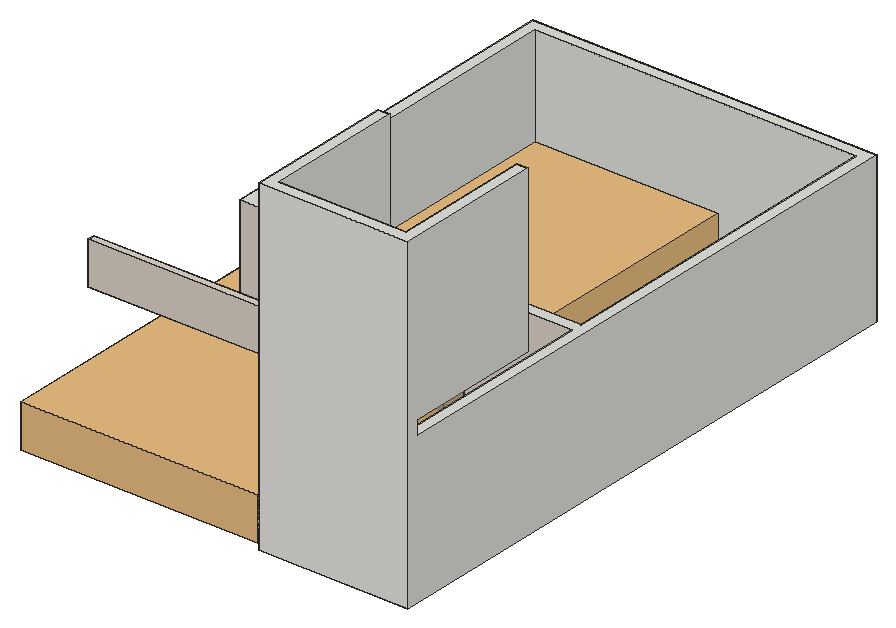
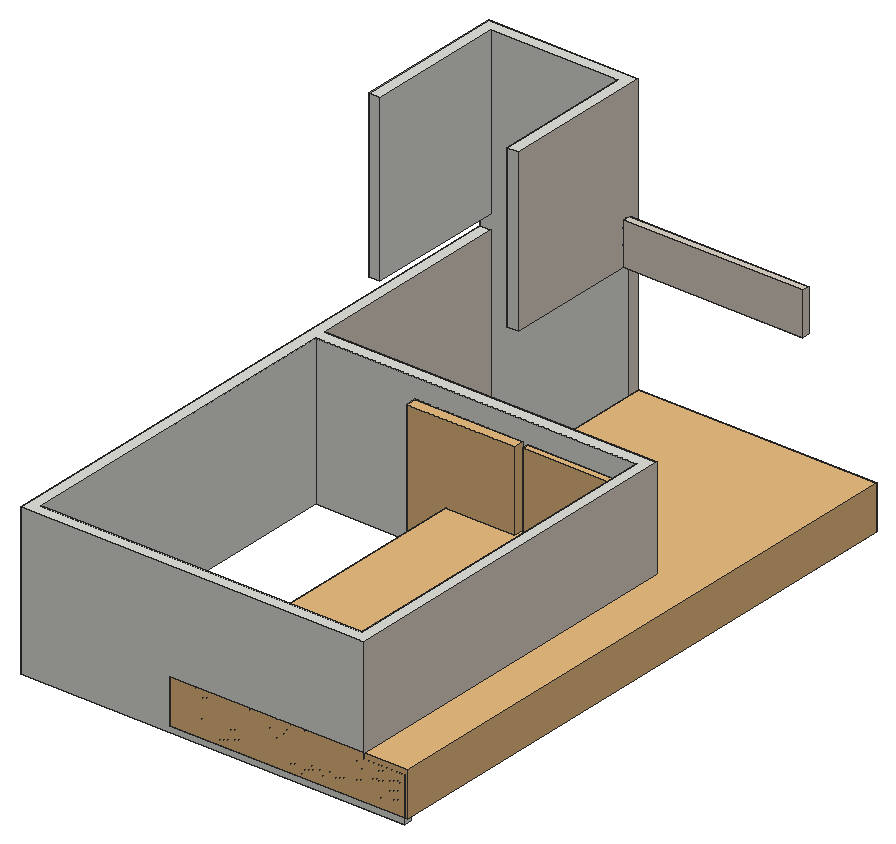
# SketchUp Ruby script. Lengths in inches.
U = 1.inch
M = Sketchup.active_model
def pt(a) = Geom::Point3d.new(a.map { |v| v * U })
def face(e, loops, mat)
  f = e.add_face(loops[0].map { |a| pt(a) })
  loops[1..].each { |l| e.add_face(l.map { |a| pt(a) }).erase! }
  f.material = f.back_material = mat if mat
  f
end
# faces: each face lists its corners as indices into pts; further lists are holes
def faces(e, pts, list, mat = nil) = list.each { |f| face(e, (f[0].is_a?(Array) ? f : [f]).map { |l| l.map { |i| pts[i] } }, mat) }
# xy, xz, yz: faces in a plane at the given z, y or x. An outline is a flat list of corners, or four numbers for a rectangle; further outlines are holes
def ring(l) = l.size == 4 ? [[l[0], l[1]], [l[2], l[1]], [l[2], l[3]], [l[0], l[3]]] : l.each_slice(2).to_a
def flat(e, list, mat, &to3) = list.each { |f| face(e, (f[0].is_a?(Array) ? f : [f]).map { |l| ring(l).map { |u, v| to3.(u, v) } }, mat) }
def xy(e, z, list, mat = nil) = flat(e, list, mat) { |x, y| [x, y, z] }
def xz(e, y, list, mat = nil) = flat(e, list, mat) { |x, z| [x, y, z] }
def yz(e, x, list, mat = nil) = flat(e, list, mat) { |y, z| [x, y, z] }
def lines(e, pts, list) = list.each { |a, b| e.add_line(pt(pts[a]), pt(pts[b])) }
# prism: a flat outline (further loops are holes) pulled along v
def prism(e, loops, v, mat = nil)
  f = face(e, loops, mat); d = Geom::Vector3d.new(v.map { |x| x * U })
  f.pushpull(f.normal.samedirection?(d) ? d.length : -d.length)
end
def box(e, o, s, mat = nil) = prism(e, [[o, [o[0] + s[0], o[1], o[2]], [o[0] + s[0], o[1] + s[1], o[2]], [o[0], o[1] + s[1], o[2]]]], [0, 0, s[2]], mat)
def at(x, y, z, deg = 0) = Geom::Transformation.translation(pt([x, y, z])) * Geom::Transformation.rotation(ORIGIN, Z_AXIS, deg.degrees)
def axes(o, x, y, z) = Geom::Transformation.new([*x, 0, *y, 0, *z, 0, *pt(o).to_a, 1])
def part(name) = M.definitions.add(name)
# library, detail: a bought-in or finely detailed component or shape, given as its bounding box
def library(name, o, s) = part(name).tap { |d| box(d.entities, o, s) }
def detail(e, o, s) = box(e.add_group.entities, o, s)
def put(e, d, t, mat = nil) = e.add_instance(d, t).tap { |i| i.material = mat if mat }
def group(e, t, mat = nil) = e.add_group.tap { |g| g.transformation = t; g.material = mat if mat }.entities
root = M.entities
M.materials.add("1755 AP K184 Brass Olive-N").color = [221, 212, 201]
M.materials.add("Antracyt").color = [44, 47, 50]
M.materials.add("[0135_DarkGray]").color = [81, 81, 81]
M.materials.add("[Carrera Marble]").color = [233, 230, 225]
M.materials.add("[Metal Seamed]").color = [15, 15, 15]
M.materials.add("[Translucent Glass Gray]").color = [128, 128, 128]
M.materials["[Translucent Glass Gray]"].alpha = 0.15
c1 = library("Group\#24",[0,0,0],[191,470.5,35])
c2 = part("หน้าต่าง3บาน")
xy(c2.entities,42.78,[[77.6875,12.74,148.55,16.68]],"Antracyt")
xy(c2.entities,43.96,[[78.87,12.74,147.37,12.74,147.37,14.71,125.72,14.71,125.72,13.13,100.52,13.13,100.52,14.71,78.87,14.71],[100.52,13.13,102.88,14.71],[123.36,13.13,125.72,14.71],[102.49,14.71,123.75,14.71,123.75,16.28,147.37,16.28,147.37,16.68,78.87,16.68,78.87,16.28,102.49,16.28]],"Antracyt")
xy(c2.entities,45.93,[[102.49,13.13,123.75,13.92],[102.49,13.92,123.75,14.71],[80.84,14.71,100.52,15.49],[125.72,14.71,145.4,15.49],[80.84,15.49,100.52,16.28],
  [125.72,15.49,145.4,16.28]],"Antracyt")
xy(c2.entities,83.09,[[102.49,13.13,123.75,13.92],[102.49,13.92,123.75,14.71],[80.84,14.71,100.52,15.49],[125.72,14.71,145.4,15.49],[80.84,15.49,100.52,16.28],
  [125.72,15.49,145.4,16.28]],"Antracyt")
xy(c2.entities,84.91,[[78.87,12.74,78.87,14.71,100.52,14.71,100.52,13.13,125.72,13.13,125.72,14.71,147.37,14.71,147.37,12.74],[100.52,13.13,125.72,14.71],[102.49,14.71,102.49,16.28,78.87,16.28,78.87,16.68,147.37,16.68,147.37,16.28,123.75,16.28,123.75,14.71],[78.87,14.71,102.49,16.28]],"Antracyt")
xy(c2.entities,86.09,[[77.6875,12.74,148.55,16.68]],"Antracyt")
xz(c2.entities,12.74,[[[77.6875,42.78,148.55,86.09],[78.87,43.96,147.37,84.91]]],"Antracyt")
xz(c2.entities,13.13,[[[100.52,43.96,125.72,84.91],[102.49,45.93,123.75,83.09]]],"Antracyt")
xz(c2.entities,13.92,[[102.49,45.93,123.75,83.09]],"Antracyt")
xz(c2.entities,14.71,[[78.87,43.96,100.52,43.96,100.52,45.93,80.84,45.93,80.84,83.09,100.52,83.09,100.52,84.91,78.87,84.91],[100.52,43.96,102.49,84.91],[102.49,43.96,123.75,45.93],[125.72,43.96,147.37,43.96,147.37,84.91,125.72,84.91,125.72,83.09,145.4,83.09,145.4,45.93,125.72,45.93],[102.49,83.09,123.75,84.91]],"Antracyt")
xz(c2.entities,15.49,[[80.84,45.93,100.52,83.09],[125.72,45.93,145.4,83.09],[80.44,82.9375,80.84,83.73]],"Antracyt")
xz(c2.entities,16.28,[[[78.87,43.96,102.49,84.91],[80.84,45.93,100.52,83.09]],[[123.75,43.96,147.37,84.91],[125.72,45.93,145.4,83.09]]],"Antracyt")
xz(c2.entities,16.68,[[[77.6875,42.78,148.55,86.09],[78.87,43.96,147.37,84.91]]],"Antracyt")
yz(c2.entities,77.6875,[[12.74,42.78,16.68,86.09]],"Antracyt")
yz(c2.entities,78.87,[[12.74,43.96,14.71,84.91],[16.28,43.96,16.68,84.91]],"Antracyt")
yz(c2.entities,80.84,[[14.71,45.93,15.49,83.09],[15.49,45.93,16.28,83.09]],"Antracyt")
yz(c2.entities,100.52,[[13.13,43.96,14.71,84.91],[14.71,45.93,15.49,83.09],[15.49,45.93,16.28,83.09]],"Antracyt")
yz(c2.entities,102.49,[[14.71,43.96,16.28,84.91],[13.13,45.93,13.92,83.09],[13.92,45.93,14.71,83.09]],"Antracyt")
yz(c2.entities,123.75,[[14.71,43.96,16.28,84.91],[13.13,45.93,13.92,83.09],[13.92,45.93,14.71,83.09]],"Antracyt")
yz(c2.entities,125.72,[[13.13,43.96,14.71,84.91],[14.71,45.93,15.49,83.09],[15.49,45.93,16.28,83.09]],"Antracyt")
yz(c2.entities,145.4,[[14.71,45.93,15.49,83.09],[15.49,45.93,16.28,83.09]],"Antracyt")
yz(c2.entities,147.37,[[12.74,43.96,14.71,84.91],[16.28,43.96,16.68,84.91]],"Antracyt")
yz(c2.entities,148.55,[[12.74,42.78,16.68,86.09]],"Antracyt")
p = [[80.44,15.49,84.91],[80.44,15.49,83.73]]
lines(c2.entities,p,[[0,1]])
c3 = part("PENTEK_RP Fineline 50S_Sliding_DoorCase_E1")
box(c3.entities,[0,0,0],[1.51,3.66,99.27],"[0135_DarkGray]")
c4 = part("PENTEK_RP Fineline 50S_SlidingDooe_Case_E2")
box(c4.entities,[0,0,0],[96.25,3.66,1.51],"[0135_DarkGray]")
c5 = part("pentek_RP Fineline 50S_SlidingDoor_Case")
put(c5.entities,c3,at(97.76,0,0))
put(c5.entities,c4,at(1.51,0,0))
put(c5.entities,c3,at(0,0,0))
put(c5.entities,c4,at(1.51,0,97.76))
c6 = part("PENTEK_RP Fineline 50S_SlidingDoor_GlazingBead_2")
box(c6.entities,[0,0,0],[0.56,0.59,94.39],"[0135_DarkGray]")
c7 = part("PENTEK_RP Fineline 50S_SlidingDoor_Glass")
box(c7.entities,[0,0,0],[46.58,0.16,94.39],"[Translucent Glass Gray]")
c8 = part("PENTEK_RP Fineline 50S_SlidingDoor_GlazingBead")
box(c8.entities,[0,0,0],[45.47,0.59,0.56],"[0135_DarkGray]")
c9 = part("PENTEK_RP Fineline 50S_SlidingDoor_Leaf_E1")
xy(c9.entities,0,[[0,0,0.93,1.97],[0.93,1.57,1.49,1.97]],"[0135_DarkGray]")
xy(c9.entities,96.25,[[0,0,0.93,0,0.93,1.57,1.49,1.57,1.49,1.97,0,1.97]],"[0135_DarkGray]")
xz(c9.entities,0,[[0,0,0.93,96.25]],"[0135_DarkGray]")
xz(c9.entities,1.57,[[0.93,0,1.49,95.32],[0.93,95.32,1.49,96.25]],"[0135_DarkGray]")
xz(c9.entities,1.97,[[0,0,1.49,96.25]],"[0135_DarkGray]")
yz(c9.entities,0,[[0,0,1.97,96.25]],"[0135_DarkGray]")
yz(c9.entities,0.93,[[0,0,1.57,0.93],[0,0.93,1.57,95.32],[0,95.32,1.57,96.25]],"[0135_DarkGray]")
yz(c9.entities,1.49,[[1.57,0,1.97,95.32],[1.57,95.32,1.97,96.25]],"[0135_DarkGray]")
c10 = part("PENTEK_RP Fineline 50S_SlidingDoor_Leaf_E2")
xy(c10.entities,0,[[0,0,0,1.57,0.56,1.57,0.56,1.97,46.02,1.97,46.02,1.57,46.58,1.57,46.58,0]],"[0135_DarkGray]")
xy(c10.entities,0.93,[[0,0,46.58,1.57]],"[0135_DarkGray]")
xy(c10.entities,1.49,[[0.56,1.57,46.02,1.97]],"[0135_DarkGray]")
xz(c10.entities,0,[[0,0,46.58,0.93]],"[0135_DarkGray]")
xz(c10.entities,1.57,[[0,0,0.56,0.93],[46.02,0,46.58,0.93],[0.56,0.93,46.02,1.49]],"[0135_DarkGray]")
xz(c10.entities,1.97,[[0.56,0,46.02,1.49]],"[0135_DarkGray]")
yz(c10.entities,0,[[0,0,1.57,0.93]],"[0135_DarkGray]")
yz(c10.entities,0.56,[[1.57,0,1.97,0.93],[1.57,0.93,1.97,1.49]],"[0135_DarkGray]")
yz(c10.entities,46.02,[[1.57,0,1.97,0.93],[1.57,0.93,1.97,1.49]],"[0135_DarkGray]")
yz(c10.entities,46.58,[[0,0,1.57,0.93]],"[0135_DarkGray]")
c11 = part("PENTEK_RP Fineline S_SlidingDoor_Leaf1")
put(c11.entities,c6,at(0.93,0,0.93))
put(c11.entities,c6,at(46.96,0,0.93))
put(c11.entities,c7,at(1.49,1.42,0.93))
put(c11.entities,c8,at(1.49,0,0.93))
put(c11.entities,c7,at(1.49,0.59,0.93))
put(c11.entities,c9,at(0,0,0))
put(c11.entities,c9,axes([48.44,0,0],[-1,0,0],[0,1,0],[0,0,1]))
put(c11.entities,c10,axes([0.93,0,96.25],[1,0,0],[0,1,0],[0,0,-1]))
put(c11.entities,c10,at(0.93,0,0))
put(c11.entities,c8,at(1.49,0,94.77))
c12 = part("PENTEK_RP Fineline 50S_SlidingDoor_Leaf2")
put(c12.entities,c7,at(1.49,1.42,0.93))
put(c12.entities,c8,at(1.49,0,94.77))
put(c12.entities,c6,at(46.96,0,0.93))
put(c12.entities,c7,at(1.49,0.59,0.93))
put(c12.entities,c6,at(0.93,0,0.93))
put(c12.entities,c9,at(0,0,0))
put(c12.entities,c9,axes([48.44,0,0],[-1,0,0],[0,1,0],[0,0,1]))
put(c12.entities,c8,at(1.49,0,0.93))
put(c12.entities,c10,axes([0.93,0,96.25],[1,0,0],[0,1,0],[0,0,-1]))
put(c12.entities,c10,at(0.93,0,0))
c13 = part("PENTEK_RP+Fineline+50S_Sliding_Door (1)")
put(c13.entities,c5,at(0,-1.88,-0.09))
put(c13.entities,c11,at(1.51,-2.27,1.42))
put(c13.entities,c12,at(49.32,-0.3,1.42))
c14 = library("Untitled",[23.5,7.18,0],[66.61,8.2,79.03])
xy(root,132,[[30.34,172.75,30.26,172.76,30.1875,172.77,30.11,172.78,29.95,172.8,29.875,172.82,29.8,172.83,29.72,172.85,29.65,172.875,29.57,172.9,29.5,172.92,29.42,172.95,29.21,173.04,29.14,173.08,29.07,173.11,28.93,173.19,28.87,173.23,28.8,173.28,28.74,173.32,28.67,173.37,28.43,173.57,28.38,173.63,28.32,173.68,28.12,173.92,28.07,173.99,28.03,174.05,27.98,174.12,27.94,174.18,27.86,174.32,27.83,174.39,27.79,174.46,27.7,174.67,27.67,174.75,27.65,174.82,27.625,174.9,27.6,174.97,27.58,175.05,27.57,175.125,27.55,175.2,27.53,175.36,27.52,175.4375,27.51,175.51,27.5,175.59,27.5,175.91,27.51,175.99,27.52,176.0625,27.53,176.14,27.55,176.3,27.57,176.375,27.58,176.45,27.6,176.53,27.625,176.6,27.65,176.68,27.67,176.75,27.7,176.83,27.79,177.04,27.83,177.11,27.86,177.18,27.94,177.32,27.98,177.38,28.03,177.45,28.07,177.51,28.12,177.58,28.32,177.82,28.38,177.87,28.43,177.93,28.67,178.13,28.74,178.18,28.8,178.22,28.87,178.27,28.93,178.31,29.07,178.39,29.14,178.42,29.21,178.46,29.42,178.55,29.5,178.58,29.57,178.6,29.65,178.625,29.72,178.65,29.8,178.67,29.875,178.68,29.95,178.7,30.11,178.72,30.1875,178.73,30.26,178.74,30.34,178.75,30.66,178.75,30.74,178.74,30.8125,178.73,30.89,178.72,31.05,178.7,31.125,178.68,31.2,178.67,31.28,178.65,31.35,178.625,31.43,178.6,31.5,178.58,31.58,178.55,31.79,178.46,31.86,178.42,31.93,178.39,32.07,178.31,32.13,178.27,32.2,178.22,32.26,178.18,32.33,178.13,32.57,177.93,32.62,177.87,32.68,177.82,32.88,177.58,32.93,177.51,32.97,177.45,33.02,177.38,33.06,177.32,33.14,177.18,33.17,177.11,33.21,177.04,33.3,176.83,33.33,176.75,33.35,176.68,33.375,176.6,33.4,176.53,33.42,176.45,33.43,176.375,33.45,176.3,33.47,176.14,33.48,176.0625,33.49,175.99,33.5,175.91,33.5,175.59,33.49,175.51,33.48,175.4375,33.47,175.36,33.45,175.2,33.43,175.125,33.42,175.05,33.4,174.97,33.375,174.9,33.35,174.82,33.33,174.75,33.3,174.67,33.21,174.46,33.17,174.39,33.14,174.32,33.06,174.18,33.02,174.12,32.97,174.05,32.93,173.99,32.88,173.92,32.68,173.68,32.62,173.63,32.57,173.57,32.33,173.37,32.26,173.32,32.2,173.28,32.13,173.23,32.07,173.19,31.93,173.11,31.86,173.08,31.79,173.04,31.58,172.95,31.5,172.92,31.43,172.9,31.35,172.875,31.28,172.85,31.2,172.83,31.125,172.82,31.05,172.8,30.89,172.78,30.8125,172.77,30.74,172.76,30.66,172.75],[100.84,172.75,100.76,172.76,100.6875,172.77,100.61,172.78,100.45,172.8,100.375,172.82,100.3,172.83,100.22,172.85,100.15,172.875,100.07,172.9,100,172.92,99.92,172.95,99.71,173.04,99.64,173.08,99.57,173.11,99.43,173.19,99.37,173.23,99.3,173.28,99.24,173.32,99.17,173.37,98.93,173.57,98.88,173.63,98.82,173.68,98.62,173.92,98.57,173.99,98.53,174.05,98.48,174.12,98.44,174.18,98.36,174.32,98.33,174.39,98.29,174.46,98.2,174.67,98.17,174.75,98.15,174.82,98.125,174.9,98.1,174.97,98.08,175.05,98.07,175.125,98.05,175.2,98.03,175.36,98.02,175.4375,98.01,175.51,98,175.59,98,175.91,98.01,175.99,98.02,176.0625,98.03,176.14,98.05,176.3,98.07,176.375,98.08,176.45,98.1,176.53,98.125,176.6,98.15,176.68,98.17,176.75,98.2,176.83,98.29,177.04,98.33,177.11,98.36,177.18,98.44,177.32,98.48,177.38,98.53,177.45,98.57,177.51,98.62,177.58,98.82,177.82,98.88,177.87,98.93,177.93,99.17,178.13,99.24,178.18,99.3,178.22,99.37,178.27,99.43,178.31,99.57,178.39,99.64,178.42,99.71,178.46,99.92,178.55,100,178.58,100.07,178.6,100.15,178.625,100.22,178.65,100.3,178.67,100.375,178.68,100.45,178.7,100.61,178.72,100.6875,178.73,100.76,178.74,100.84,178.75,101.16,178.75,101.24,178.74,101.3125,178.73,101.39,178.72,101.55,178.7,101.625,178.68,101.7,178.67,101.78,178.65,101.85,178.625,101.93,178.6,102,178.58,102.08,178.55,102.29,178.46,102.36,178.42,102.43,178.39,102.57,178.31,102.63,178.27,102.7,178.22,102.76,178.18,102.83,178.13,103.07,177.93,103.12,177.87,103.18,177.82,103.38,177.58,103.43,177.51,103.47,177.45,103.52,177.38,103.56,177.32,103.64,177.18,103.67,177.11,103.71,177.04,103.8,176.83,103.83,176.75,103.85,176.68,103.875,176.6,103.9,176.53,103.92,176.45,103.93,176.375,103.95,176.3,103.97,176.14,103.98,176.0625,103.99,175.99,104,175.91,104,175.59,103.99,175.51,103.98,175.4375,103.97,175.36,103.95,175.2,103.93,175.125,103.92,175.05,103.9,174.97,103.875,174.9,103.85,174.82,103.83,174.75,103.8,174.67,103.71,174.46,103.67,174.39,103.64,174.32,103.56,174.18,103.52,174.12,103.47,174.05,103.43,173.99,103.38,173.92,103.18,173.68,103.12,173.63,103.07,173.57,102.83,173.37,102.76,173.32,102.7,173.28,102.63,173.23,102.57,173.19,102.43,173.11,102.36,173.08,102.29,173.04,102.08,172.95,102,172.92,101.93,172.9,101.85,172.875,101.78,172.85,101.7,172.83,101.625,172.82,101.55,172.8,101.39,172.78,101.3125,172.77,101.24,172.76,101.16,172.75],[30.34,226.5,30.26,226.51,30.1875,226.52,30.11,226.53,29.95,226.55,29.875,226.57,29.8,226.58,29.72,226.6,29.65,226.625,29.57,226.65,29.5,226.67,29.42,226.7,29.21,226.79,29.14,226.83,29.07,226.86,28.93,226.94,28.87,226.98,28.8,227.03,28.74,227.07,28.67,227.12,28.43,227.32,28.38,227.38,28.32,227.43,28.12,227.67,28.07,227.74,28.03,227.8,27.98,227.87,27.94,227.93,27.86,228.07,27.83,228.14,27.79,228.21,27.7,228.42,27.67,228.5,27.65,228.57,27.625,228.65,27.6,228.72,27.58,228.8,27.57,228.875,27.55,228.95,27.53,229.11,27.52,229.1875,27.51,229.26,27.5,229.34,27.5,229.66,27.51,229.74,27.52,229.8125,27.53,229.89,27.55,230.05,27.57,230.125,27.58,230.2,27.6,230.28,27.625,230.35,27.65,230.43,27.67,230.5,27.7,230.58,27.79,230.79,27.83,230.86,27.86,230.93,27.94,231.07,27.98,231.13,28.03,231.2,28.07,231.26,28.12,231.33,28.32,231.57,28.38,231.62,28.43,231.68,28.67,231.88,28.74,231.93,28.8,231.97,28.87,232.02,28.93,232.06,29.07,232.14,29.14,232.17,29.21,232.21,29.42,232.3,29.5,232.33,29.57,232.35,29.65,232.375,29.72,232.4,29.8,232.42,29.875,232.43,29.95,232.45,30.11,232.47,30.1875,232.48,30.26,232.49,30.34,232.5,30.66,232.5,30.74,232.49,30.8125,232.48,30.89,232.47,31.05,232.45,31.125,232.43,31.2,232.42,31.28,232.4,31.35,232.375,31.43,232.35,31.5,232.33,31.58,232.3,31.79,232.21,31.86,232.17,31.93,232.14,32.07,232.06,32.13,232.02,32.2,231.97,32.26,231.93,32.33,231.88,32.57,231.68,32.62,231.62,32.68,231.57,32.88,231.33,32.93,231.26,32.97,231.2,33.02,231.13,33.06,231.07,33.14,230.93,33.17,230.86,33.21,230.79,33.3,230.58,33.33,230.5,33.35,230.43,33.375,230.35,33.4,230.28,33.42,230.2,33.43,230.125,33.45,230.05,33.47,229.89,33.48,229.8125,33.49,229.74,33.5,229.66,33.5,229.34,33.49,229.26,33.48,229.1875,33.47,229.11,33.45,228.95,33.43,228.875,33.42,228.8,33.4,228.72,33.375,228.65,33.35,228.57,33.33,228.5,33.3,228.42,33.21,228.21,33.17,228.14,33.14,228.07,33.06,227.93,33.02,227.87,32.97,227.8,32.93,227.74,32.88,227.67,32.68,227.43,32.62,227.38,32.57,227.32,32.33,227.12,32.26,227.07,32.2,227.03,32.13,226.98,32.07,226.94,31.93,226.86,31.86,226.83,31.79,226.79,31.58,226.7,31.5,226.67,31.43,226.65,31.35,226.625,31.28,226.6,31.2,226.58,31.125,226.57,31.05,226.55,30.89,226.53,30.8125,226.52,30.74,226.51,30.66,226.5],[100.84,226.5,100.76,226.51,100.6875,226.52,100.61,226.53,100.45,226.55,100.375,226.57,100.3,226.58,100.22,226.6,100.15,226.625,100.07,226.65,100,226.67,99.92,226.7,99.71,226.79,99.64,226.83,99.57,226.86,99.43,226.94,99.37,226.98,99.3,227.03,99.24,227.07,99.17,227.12,98.93,227.32,98.88,227.38,98.82,227.43,98.62,227.67,98.57,227.74,98.53,227.8,98.48,227.87,98.44,227.93,98.36,228.07,98.33,228.14,98.29,228.21,98.2,228.42,98.17,228.5,98.15,228.57,98.125,228.65,98.1,228.72,98.08,228.8,98.07,228.875,98.05,228.95,98.03,229.11,98.02,229.1875,98.01,229.26,98,229.34,98,229.66,98.01,229.74,98.02,229.8125,98.03,229.89,98.05,230.05,98.07,230.125,98.08,230.2,98.1,230.28,98.125,230.35,98.15,230.43,98.17,230.5,98.2,230.58,98.29,230.79,98.33,230.86,98.36,230.93,98.44,231.07,98.48,231.13,98.53,231.2,98.57,231.26,98.62,231.33,98.82,231.57,98.88,231.62,98.93,231.68,99.17,231.88,99.24,231.93,99.3,231.97,99.37,232.02,99.43,232.06,99.57,232.14,99.64,232.17,99.71,232.21,99.92,232.3,100,232.33,100.07,232.35,100.15,232.375,100.22,232.4,100.3,232.42,100.375,232.43,100.45,232.45,100.61,232.47,100.6875,232.48,100.76,232.49,100.84,232.5,101.16,232.5,101.24,232.49,101.3125,232.48,101.39,232.47,101.55,232.45,101.625,232.43,101.7,232.42,101.78,232.4,101.85,232.375,101.93,232.35,102,232.33,102.08,232.3,102.29,232.21,102.36,232.17,102.43,232.14,102.57,232.06,102.63,232.02,102.7,231.97,102.76,231.93,102.83,231.88,103.07,231.68,103.12,231.62,103.18,231.57,103.38,231.33,103.43,231.26,103.47,231.2,103.52,231.13,103.56,231.07,103.64,230.93,103.67,230.86,103.71,230.79,103.8,230.58,103.83,230.5,103.85,230.43,103.875,230.35,103.9,230.28,103.92,230.2,103.93,230.125,103.95,230.05,103.97,229.89,103.98,229.8125,103.99,229.74,104,229.66,104,229.34,103.99,229.26,103.98,229.1875,103.97,229.11,103.95,228.95,103.93,228.875,103.92,228.8,103.9,228.72,103.875,228.65,103.85,228.57,103.83,228.5,103.8,228.42,103.71,228.21,103.67,228.14,103.64,228.07,103.56,227.93,103.52,227.87,103.47,227.8,103.43,227.74,103.38,227.67,103.18,227.43,103.12,227.38,103.07,227.32,102.83,227.12,102.76,227.07,102.7,227.03,102.63,226.98,102.57,226.94,102.43,226.86,102.36,226.83,102.29,226.79,102.08,226.7,102,226.67,101.93,226.65,101.85,226.625,101.78,226.6,101.7,226.58,101.625,226.57,101.55,226.55,101.39,226.53,101.3125,226.52,101.24,226.51,101.16,226.5],[30.34,329,30.26,329.01,30.1875,329.02,30.11,329.03,29.95,329.05,29.875,329.07,29.8,329.08,29.72,329.1,29.65,329.125,29.57,329.15,29.5,329.17,29.42,329.2,29.21,329.29,29.14,329.33,29.07,329.36,28.93,329.44,28.87,329.48,28.8,329.53,28.74,329.57,28.67,329.62,28.43,329.82,28.38,329.88,28.32,329.93,28.12,330.17,28.07,330.24,28.03,330.3,27.98,330.37,27.94,330.43,27.86,330.57,27.83,330.64,27.79,330.71,27.7,330.92,27.67,331,27.65,331.07,27.625,331.15,27.6,331.22,27.58,331.3,27.57,331.375,27.55,331.45,27.53,331.61,27.52,331.6875,27.51,331.76,27.5,331.84,27.5,332.16,27.51,332.24,27.52,332.3125,27.53,332.39,27.55,332.55,27.57,332.625,27.58,332.7,27.6,332.78,27.625,332.85,27.65,332.93,27.67,333,27.7,333.08,27.79,333.29,27.83,333.36,27.86,333.43,27.94,333.57,27.98,333.63,28.03,333.7,28.07,333.76,28.12,333.83,28.32,334.07,28.38,334.12,28.43,334.18,28.67,334.38,28.74,334.43,28.8,334.47,28.87,334.52,28.93,334.56,29.07,334.64,29.14,334.67,29.21,334.71,29.42,334.8,29.5,334.83,29.57,334.85,29.65,334.875,29.72,334.9,29.8,334.92,29.875,334.93,29.95,334.95,30.11,334.97,30.1875,334.98,30.26,334.99,30.34,335,30.66,335,30.74,334.99,30.8125,334.98,30.89,334.97,31.05,334.95,31.125,334.93,31.2,334.92,31.28,334.9,31.35,334.875,31.43,334.85,31.5,334.83,31.58,334.8,31.79,334.71,31.86,334.67,31.93,334.64,32.07,334.56,32.13,334.52,32.2,334.47,32.26,334.43,32.33,334.38,32.57,334.18,32.62,334.12,32.68,334.07,32.88,333.83,32.93,333.76,32.97,333.7,33.02,333.63,33.06,333.57,33.14,333.43,33.17,333.36,33.21,333.29,33.3,333.08,33.33,333,33.35,332.93,33.375,332.85,33.4,332.78,33.42,332.7,33.43,332.625,33.45,332.55,33.47,332.39,33.48,332.3125,33.49,332.24,33.5,332.16,33.5,331.84,33.49,331.76,33.48,331.6875,33.47,331.61,33.45,331.45,33.43,331.375,33.42,331.3,33.4,331.22,33.375,331.15,33.35,331.07,33.33,331,33.3,330.92,33.21,330.71,33.17,330.64,33.14,330.57,33.06,330.43,33.02,330.37,32.97,330.3,32.93,330.24,32.88,330.17,32.68,329.93,32.62,329.88,32.57,329.82,32.33,329.62,32.26,329.57,32.2,329.53,32.13,329.48,32.07,329.44,31.93,329.36,31.86,329.33,31.79,329.29,31.58,329.2,31.5,329.17,31.43,329.15,31.35,329.125,31.28,329.1,31.2,329.08,31.125,329.07,31.05,329.05,30.89,329.03,30.8125,329.02,30.74,329.01,30.66,329],
  [30.34,431.5,30.26,431.51,30.1875,431.52,30.11,431.53,29.95,431.55,29.875,431.57,29.8,431.58,29.72,431.6,29.65,431.625,29.57,431.65,29.5,431.67,29.42,431.7,29.21,431.79,29.14,431.83,29.07,431.86,28.93,431.94,28.87,431.98,28.8,432.03,28.74,432.07,28.67,432.12,28.43,432.32,28.38,432.38,28.32,432.43,28.12,432.67,28.07,432.74,28.03,432.8,27.98,432.87,27.94,432.93,27.86,433.07,27.83,433.14,27.79,433.21,27.7,433.42,27.67,433.5,27.65,433.57,27.625,433.65,27.6,433.72,27.58,433.8,27.57,433.875,27.55,433.95,27.53,434.11,27.52,434.1875,27.51,434.26,27.5,434.34,27.5,434.66,27.51,434.74,27.52,434.8125,27.53,434.89,27.55,435.05,27.57,435.125,27.58,435.2,27.6,435.28,27.625,435.35,27.65,435.43,27.67,435.5,27.7,435.58,27.79,435.79,27.83,435.86,27.86,435.93,27.94,436.07,27.98,436.13,28.03,436.2,28.07,436.26,28.12,436.33,28.32,436.57,28.38,436.62,28.43,436.68,28.67,436.88,28.74,436.93,28.8,436.97,28.87,437.02,28.93,437.06,29.07,437.14,29.14,437.17,29.21,437.21,29.42,437.3,29.5,437.33,29.57,437.35,29.65,437.375,29.72,437.4,29.8,437.42,29.875,437.43,29.95,437.45,30.11,437.47,30.1875,437.48,30.26,437.49,30.34,437.5,30.66,437.5,30.74,437.49,30.8125,437.48,30.89,437.47,31.05,437.45,31.125,437.43,31.2,437.42,31.28,437.4,31.35,437.375,31.43,437.35,31.5,437.33,31.58,437.3,31.79,437.21,31.86,437.17,31.93,437.14,32.07,437.06,32.13,437.02,32.2,436.97,32.26,436.93,32.33,436.88,32.57,436.68,32.62,436.62,32.68,436.57,32.88,436.33,32.93,436.26,32.97,436.2,33.02,436.13,33.06,436.07,33.14,435.93,33.17,435.86,33.21,435.79,33.3,435.58,33.33,435.5,33.35,435.43,33.375,435.35,33.4,435.28,33.42,435.2,33.43,435.125,33.45,435.05,33.47,434.89,33.48,434.8125,33.49,434.74,33.5,434.66,33.5,434.34,33.49,434.26,33.48,434.1875,33.47,434.11,33.45,433.95,33.43,433.875,33.42,433.8,33.4,433.72,33.375,433.65,33.35,433.57,33.33,433.5,33.3,433.42,33.21,433.21,33.17,433.14,33.14,433.07,33.06,432.93,33.02,432.87,32.97,432.8,32.93,432.74,32.88,432.67,32.68,432.43,32.62,432.38,32.57,432.32,32.33,432.12,32.26,432.07,32.2,432.03,32.13,431.98,32.07,431.94,31.93,431.86,31.86,431.83,31.79,431.79,31.58,431.7,31.5,431.67,31.43,431.65,31.35,431.625,31.28,431.6,31.2,431.58,31.125,431.57,31.05,431.55,30.89,431.53,30.8125,431.52,30.74,431.51,30.66,431.5],[30.34,534,30.26,534.01,30.1875,534.02,30.11,534.03,29.95,534.05,29.875,534.07,29.8,534.08,29.72,534.1,29.65,534.125,29.57,534.15,29.5,534.17,29.42,534.2,29.21,534.29,29.14,534.33,29.07,534.36,28.93,534.44,28.87,534.48,28.8,534.53,28.74,534.57,28.67,534.62,28.43,534.82,28.38,534.88,28.32,534.93,28.12,535.17,28.07,535.24,28.03,535.3,27.98,535.37,27.94,535.43,27.86,535.57,27.83,535.64,27.79,535.71,27.7,535.92,27.67,536,27.65,536.07,27.625,536.15,27.6,536.22,27.58,536.3,27.57,536.375,27.55,536.45,27.53,536.61,27.52,536.6875,27.51,536.76,27.5,536.84,27.5,537.16,27.51,537.24,27.52,537.3125,27.53,537.39,27.55,537.55,27.57,537.625,27.58,537.7,27.6,537.78,27.625,537.85,27.65,537.93,27.67,538,27.7,538.08,27.79,538.29,27.83,538.36,27.86,538.43,27.94,538.57,27.98,538.63,28.03,538.7,28.07,538.76,28.12,538.83,28.32,539.07,28.38,539.12,28.43,539.18,28.67,539.38,28.74,539.43,28.8,539.47,28.87,539.52,28.93,539.56,29.07,539.64,29.14,539.67,29.21,539.71,29.42,539.8,29.5,539.83,29.57,539.85,29.65,539.875,29.72,539.9,29.8,539.92,29.875,539.93,29.95,539.95,30.11,539.97,30.1875,539.98,30.26,539.99,30.34,540,30.66,540,30.74,539.99,30.8125,539.98,30.89,539.97,31.05,539.95,31.125,539.93,31.2,539.92,31.28,539.9,31.35,539.875,31.43,539.85,31.5,539.83,31.58,539.8,31.79,539.71,31.86,539.67,31.93,539.64,32.07,539.56,32.13,539.52,32.2,539.47,32.26,539.43,32.33,539.38,32.57,539.18,32.62,539.12,32.68,539.07,32.88,538.83,32.93,538.76,32.97,538.7,33.02,538.63,33.06,538.57,33.14,538.43,33.17,538.36,33.21,538.29,33.3,538.08,33.33,538,33.35,537.93,33.375,537.85,33.4,537.78,33.42,537.7,33.43,537.625,33.45,537.55,33.47,537.39,33.48,537.3125,33.49,537.24,33.5,537.16,33.5,536.84,33.49,536.76,33.48,536.6875,33.47,536.61,33.45,536.45,33.43,536.375,33.42,536.3,33.4,536.22,33.375,536.15,33.35,536.07,33.33,536,33.3,535.92,33.21,535.71,33.17,535.64,33.14,535.57,33.06,535.43,33.02,535.37,32.97,535.3,32.93,535.24,32.88,535.17,32.68,534.93,32.62,534.88,32.57,534.82,32.33,534.62,32.26,534.57,32.2,534.53,32.13,534.48,32.07,534.44,31.93,534.36,31.86,534.33,31.79,534.29,31.58,534.2,31.5,534.17,31.43,534.15,31.35,534.125,31.28,534.1,31.2,534.08,31.125,534.07,31.05,534.05,30.89,534.03,30.8125,534.02,30.74,534.01,30.66,534]])
put(root,c1,at(12,84.5,143),"[Metal Seamed]")
g1 = group(root,at(47,261,138))
xy(g1,0,[[156,-176,156,-167,267,-167,267,0,180,0,180,9,267,9,267,285,9,285,9,9,108,9,108,0,0,0,0,288,-33,288,-33,294,276,294,276,-176]])
xy(g1,30,[[30,0,90,9]])
xy(g1,36,[[-33,288,0,294]])
xy(g1,96,[[30,0,90,9],[108,0,180,9]])
xy(g1,120,[[[267,-167,276,-167,276,294,0,294,0,0,267,0],[9,9,267,285]]])
xy(g1,132,[[267,-167,276,-56]])
xy(g1,135,[[156,-167,165,-56]])
xy(g1,264,[[156,-176,276,-176,276,-56,267,-56,267,-167,165,-167,165,-56,156,-56]])
xz(g1,-176,[[156,0,276,264]],"[Carrera Marble]")
xz(g1,-167,[[156,0,156,135,165,135,165,264,267,264,267,132,276,132,276,120,267,120,267,0]])
xz(g1,-56,[[267,132,276,264],[156,135,165,264]])
xz(g1,0,[[[0,0,108,0,108,96,180,96,180,0,267,0,267,120,0,120],[30,30,90,96]]],"1755 AP K184 Brass Olive-N")
xz(g1,9,[[[9,0,9,120,267,120,267,0,180,0,180,96,108,96,108,0],[30,30,90,96]]])
xz(g1,285,[[9,0,267,120]])
xz(g1,288,[[-33,0,0,36]])
xz(g1,294,[[-33,0,-33,36,0,36,0,120,276,120,276,0]])
yz(g1,-33,[[288,0,294,36]])
yz(g1,0,[[0,0,0,120,294,120,294,36,288,36,288,0]],"1755 AP K184 Brass Olive-N")
yz(g1,9,[[9,0,285,120]])
yz(g1,30,[[0,30,9,96]])
yz(g1,90,[[0,30,9,96]])
yz(g1,108,[[0,0,9,96]])
yz(g1,156,[[-176,0,-176,264,-56,264,-56,135,-167,135,-167,0]],"1755 AP K184 Brass Olive-N")
yz(g1,165,[[-167,135,-56,264]])
yz(g1,180,[[0,0,9,96]])
yz(g1,267,[[9,0,285,120],[-167,132,-56,264]])
yz(g1,267,[[-167,0,0,120]],"1755 AP K184 Brass Olive-N")
yz(g1,276,[[-176,0,294,0,294,120,-167,120,-167,132,-56,132,-56,264,-176,264]])
put(g1,c2,axes([-36.375,-11.24,-35.2],[0.8544,0,0],[0,1,0],[0,0,1.524]))
put(g1,c13,axes([108,2.77,0.09],[0.72528,0,0],[0,1,0],[0,0,0.96704]))
put(g1,c14,axes([70.15,1.82,0],[1.2987,0,0],[0,1,0],[0,0,1.31]))
put(g1,c14,axes([2.89,4.44,26.56],[1.03545,0,0],[0,0.67,0],[0,0,0.96547]))
g2 = group(g1,at(156,-167,135),"1755 AP K184 Brass Olive-N")
box(g2,[-144,0,0],[144,6,34])
